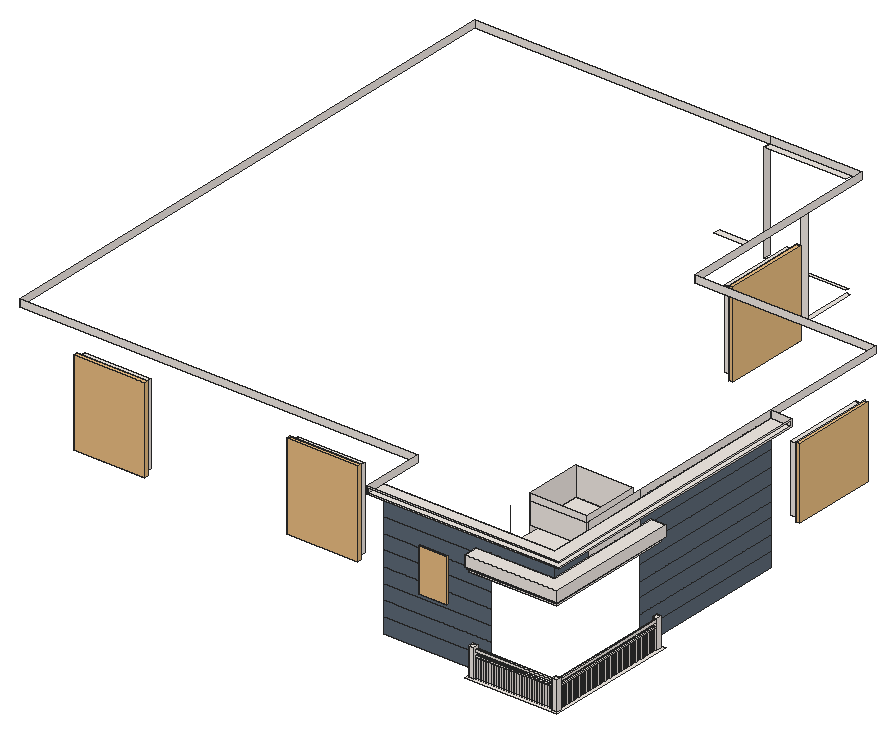
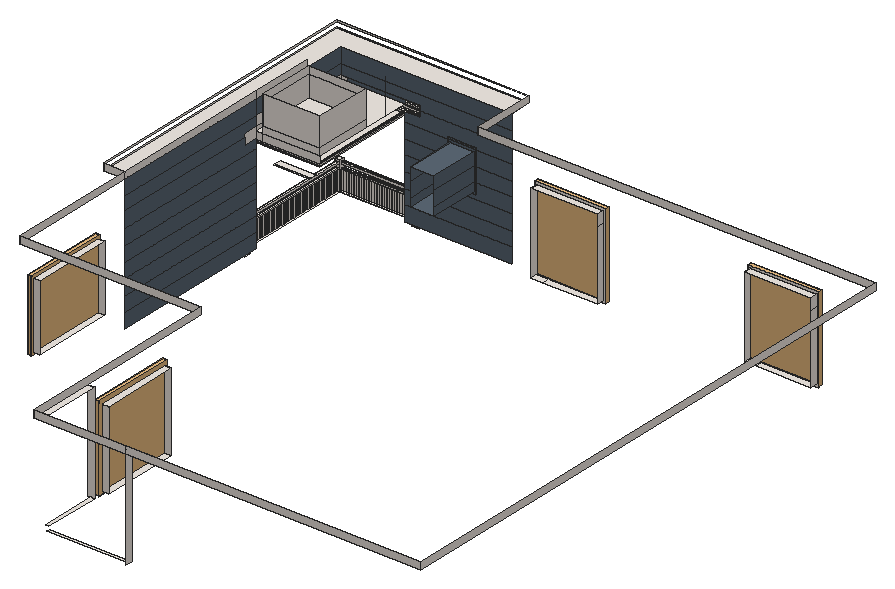
# SketchUp Ruby script. Lengths in inches.
U = 1.inch
M = Sketchup.active_model
def pt(a) = Geom::Point3d.new(a.map { |v| v * U })
def face(e, loops, mat)
  f = e.add_face(loops[0].map { |a| pt(a) })
  loops[1..].each { |l| e.add_face(l.map { |a| pt(a) }).erase! }
  f.material = f.back_material = mat if mat
  f
end
# faces: each face lists its corners as indices into pts; further lists are holes
def faces(e, pts, list, mat = nil) = list.each { |f| face(e, (f[0].is_a?(Array) ? f : [f]).map { |l| l.map { |i| pts[i] } }, mat) }
# xy, xz, yz: faces in a plane at the given z, y or x. An outline is a flat list of corners, or four numbers for a rectangle; further outlines are holes
def ring(l) = l.size == 4 ? [[l[0], l[1]], [l[2], l[1]], [l[2], l[3]], [l[0], l[3]]] : l.each_slice(2).to_a
def flat(e, list, mat, &to3) = list.each { |f| face(e, (f[0].is_a?(Array) ? f : [f]).map { |l| ring(l).map { |u, v| to3.(u, v) } }, mat) }
def xy(e, z, list, mat = nil) = flat(e, list, mat) { |x, y| [x, y, z] }
def xz(e, y, list, mat = nil) = flat(e, list, mat) { |x, z| [x, y, z] }
def yz(e, x, list, mat = nil) = flat(e, list, mat) { |y, z| [x, y, z] }
def lines(e, pts, list) = list.each { |a, b| e.add_line(pt(pts[a]), pt(pts[b])) }
# prism: a flat outline (further loops are holes) pulled along v
def prism(e, loops, v, mat = nil)
  f = face(e, loops, mat); d = Geom::Vector3d.new(v.map { |x| x * U })
  f.pushpull(f.normal.samedirection?(d) ? d.length : -d.length)
end
def box(e, o, s, mat = nil) = prism(e, [[o, [o[0] + s[0], o[1], o[2]], [o[0] + s[0], o[1] + s[1], o[2]], [o[0], o[1] + s[1], o[2]]]], [0, 0, s[2]], mat)
def at(x, y, z, deg = 0) = Geom::Transformation.translation(pt([x, y, z])) * Geom::Transformation.rotation(ORIGIN, Z_AXIS, deg.degrees)
def axes(o, x, y, z) = Geom::Transformation.new([*x, 0, *y, 0, *z, 0, *pt(o).to_a, 1])
def part(name) = M.definitions.add(name)
# library, detail: a bought-in or finely detailed component or shape, given as its bounding box
def library(name, o, s) = part(name).tap { |d| box(d.entities, o, s) }
def detail(e, o, s) = box(e.add_group.entities, o, s)
def put(e, d, t, mat = nil) = e.add_instance(d, t).tap { |i| i.material = mat if mat }
def group(e, t, mat = nil) = e.add_group.tap { |g| g.transformation = t; g.material = mat if mat }.entities
root = M.entities
M.materials.add("D01_Frost_White").color = [242, 235, 229]
M.materials.add("Denim_03_1K").color = [93, 106, 119]
c1 = library("mesh-163",[-551.08,-704.17,-20.03],[1929.24,1401.85,86.96])
c2 = part("Group11")
put(c2.entities,c1,at(0,0,0))
xy(root,258,[[[426,6,504,6,504,120,492,120,492,114,498,114,498,12,432,12,432,18,426,18],[498,8,502,12],[498,114,502,118],[428,8,432,12],[477.804,9.471,478.204,10.971],[475.655,9.471,476.055,10.971],[473.505,9.471,473.905,10.971],[471.356,9.471,471.756,10.971],[469.206,9.471,469.606,10.971],[467.057,9.471,467.457,10.971],[464.908,9.471,465.308,10.971],[462.758,9.471,463.158,10.971],[460.609,9.471,461.009,10.971],[458.459,9.471,458.859,10.971],[456.31,9.471,456.71,10.971],[454.16,9.471,454.56,10.971],[452.011,9.471,452.411,10.971],[449.862,9.471,450.262,10.971],[447.712,9.471,448.112,10.971],[445.563,9.471,445.963,10.971],[443.413,9.471,443.813,10.971],[441.264,9.471,441.664,10.971],[439.115,9.471,439.515,10.971],[432.666,9.471,433.066,10.971],[434.816,9.471,435.216,10.971],[436.965,9.471,437.365,10.971],[499.533,113.2,500.936,113.6],[499.533,110.689,500.936,111.089],[499.533,108.177,500.936,108.577],[499.533,105.666,500.936,106.066],[499.533,100.643,500.936,101.043],[499.533,103.154,500.936,103.554],[499.533,98.131,500.936,98.531]]],"D01_Frost_White")
xy(root,258.028,[[479.954,9.471,480.354,10.971],[482.103,9.471,482.503,10.971],[484.252,9.471,484.652,10.971],[486.402,9.471,486.802,10.971],[488.551,9.471,488.951,10.971],
  [490.701,9.471,491.101,10.971],[492.85,9.471,493.25,10.971],[495,9.471,495.4,10.971],[497.149,9.471,497.549,10.971],[499.533,12.739,500.936,13.139],
  [499.533,15.251,500.936,15.651],[499.533,17.762,500.936,18.162],[499.533,20.274,500.936,20.674],[499.533,22.785,500.936,23.185],[499.533,25.297,500.936,25.697],
  [499.533,27.808,500.936,28.208],[499.533,30.32,500.936,30.72],[499.533,32.831,500.936,33.231],[499.533,35.343,500.936,35.743],[499.533,37.854,500.936,38.254],
  [499.533,40.366,500.936,40.766],[499.533,42.877,500.936,43.277],[499.533,45.389,500.936,45.789],[499.533,47.9,500.936,48.3],[499.533,50.412,500.936,50.812],
  [499.533,52.923,500.936,53.323],[499.533,55.435,500.936,55.835],[499.533,57.947,500.936,58.347],[499.533,60.458,500.936,60.858],[499.533,62.97,500.936,63.37],
  [499.533,65.481,500.936,65.881],[499.533,67.993,500.936,68.393],[499.533,70.504,500.936,70.904],[499.533,73.016,500.936,73.416],[499.533,75.527,500.936,75.927],
  [499.533,78.039,500.936,78.439],[499.533,80.55,500.936,80.95],[499.533,83.062,500.936,83.462],[499.533,85.573,500.936,85.973],[499.533,88.085,500.936,88.485],
  [499.533,90.596,500.936,90.996],[499.533,93.108,500.936,93.508],[499.533,95.619,500.936,96.019]],"D01_Frost_White")
xy(root,274.664,[[[432,9.204,498,11.204],[432.666,9.471,433.066,10.971],[434.816,9.471,435.216,10.971],[436.965,9.471,437.365,10.971],[439.115,9.471,439.515,10.971],[441.264,9.471,441.664,10.971],[443.413,9.471,443.813,10.971],[445.563,9.471,445.963,10.971],[447.712,9.471,448.112,10.971],[449.862,9.471,450.262,10.971],[452.011,9.471,452.411,10.971],[454.16,9.471,454.56,10.971],[456.31,9.471,456.71,10.971],[458.459,9.471,458.859,10.971],[460.609,9.471,461.009,10.971],[462.758,9.471,463.158,10.971],[464.908,9.471,465.308,10.971],[467.057,9.471,467.457,10.971],[469.206,9.471,469.606,10.971],[471.356,9.471,471.756,10.971],[473.505,9.471,473.905,10.971],[475.655,9.471,476.055,10.971],[477.804,9.471,478.204,10.971],[479.954,9.471,480.354,10.971],[482.103,9.471,482.503,10.971],[484.252,9.471,484.652,10.971],[486.402,9.471,486.802,10.971],[488.551,9.471,488.951,10.971],[490.701,9.471,491.101,10.971],[492.85,9.471,493.25,10.971],[495,9.471,495.4,10.971],[497.149,9.471,497.549,10.971]],[[499.158,12,501.158,114],[499.533,12.739,500.936,13.139],[499.533,15.251,500.936,15.651],[499.533,17.762,500.936,18.162],[499.533,20.274,500.936,20.674],[499.533,22.785,500.936,23.185],[499.533,25.297,500.936,25.697],[499.533,27.808,500.936,28.208],[499.533,30.32,500.936,30.72],[499.533,32.831,500.936,33.231],[499.533,35.343,500.936,35.743],[499.533,37.854,500.936,38.254],[499.533,40.366,500.936,40.766],[499.533,42.877,500.936,43.277],[499.533,45.389,500.936,45.789],[499.533,47.9,500.936,48.3],[499.533,50.412,500.936,50.812],[499.533,52.923,500.936,53.323],[499.533,55.435,500.936,55.835],[499.533,57.947,500.936,58.347],[499.533,60.458,500.936,60.858],[499.533,62.97,500.936,63.37],[499.533,65.481,500.936,65.881],[499.533,67.993,500.936,68.393],[499.533,70.504,500.936,70.904],[499.533,73.016,500.936,73.416],[499.533,75.527,500.936,75.927],[499.533,78.039,500.936,78.439],[499.533,80.55,500.936,80.95],[499.533,83.062,500.936,83.462],[499.533,85.573,500.936,85.973],[499.533,88.085,500.936,88.485],[499.533,90.596,500.936,90.996],[499.533,93.108,500.936,93.508],[499.533,95.619,500.936,96.019],[499.533,98.131,500.936,98.531],[499.533,100.643,500.936,101.043],[499.533,103.154,500.936,103.554],[499.533,105.666,500.936,106.066],[499.533,108.177,500.936,108.577],[499.533,110.689,500.936,111.089],[499.533,113.2,500.936,113.6]],[499.155,12.739,499.158,13.139]],"D01_Frost_White")
xy(root,275.664,[[432,9.204,498,11.204],[499.158,12,501.158,114]],"D01_Frost_White")
xy(root,278.282,[[432,9.204,498,11.204],[499.158,12,501.158,114]],"D01_Frost_White")
xy(root,280.282,[[432,9.204,498,11.204],[499.158,12,501.158,114]],"D01_Frost_White")
xy(root,282,[[428,8,432,12],[498,8,502,12],[498,114,502,118]],"D01_Frost_White")
xy(root,284,[[62,54,108,60],[108,54,118,60],[242,54,288,60],[288,54,298,60],[486,275,492,343]],"D01_Frost_White")
xy(root,285,[[333,396,339,462]],"D01_Frost_White")
xy(root,288,[[333,477,336,525],[261,528,330,531]],"D01_Frost_White")
xy(root,302,[[380,18,400,60]],"Denim_03_1K")
xy(root,332.2,[[380,18,400,60]],"Denim_03_1K")
xy(root,333,[[441,108,471,114],[441,114,471,115.5],[264,471,294,477]],"D01_Frost_White")
xy(root,336,[[[444,12,498,102],[486,21.031,492,60]],[486,21.031,492,54],[486,29.003,492,60]],"D01_Frost_White")
xy(root,338,[[[428,8,428,16,440,16,440,106,494,106,494,118,502,118,502,8],[430,10,500,10,500,116,496,116,496,104,442,104,442,14,430,14]],[[430,10,430,14,442,14,442,104,496,104,496,116,500,116,500,10],[444,12,498,102]]],"D01_Frost_White")
xy(root,340,[[[427,7,427,17,439,17,439,107,493,107,493,119,503,119,503,7],[428,8,502,8,502,118,494,118,494,106,440,106,440,16,428,16]],[486,275,492,343]],"D01_Frost_White")
xy(root,342,[[[426,6,426,18,438,18,438,108,492,108,492,120,504,120,504,6],[427,7,503,7,503,119,493,119,493,107,439,107,439,17,427,17]],[486,54,492,60]],"D01_Frost_White")
xy(root,348,[[438,18,438,108,492,108,492,60,486,60,486,18],[486,18,492,54],[486,54,492,60]],"D01_Frost_White")
xy(root,351,[[426,6,504,6,504,120,492,120,492,18,426,18],[333,396,339,462]],"D01_Frost_White")
xy(root,352,[[62,54,118,60],[242,54,298,60]],"D01_Frost_White")
xy(root,354,[[438,60,486,108]],"D01_Frost_White")
xy(root,372,[[348,0,348,18,492,18,492,246,510,246,510,0],[333,477,339,525],[261,528,330,534]],"D01_Frost_White")
xz(root,0,[[348,372,510,372,510,373,349,373,349,377,510,377,510,378,348,378]],"D01_Frost_White")
xz(root,6,[[426,342,504,351]],"D01_Frost_White")
xz(root,7,[[427,340,503,342]],"D01_Frost_White")
xz(root,8,[[428,258,432,282],[498,258,502,282],[428,338,502,340]],"D01_Frost_White")
xz(root,9.204,[[432,274.664,498,275.664],[432,278.282,498,280.282]],"D01_Frost_White")
xz(root,9.471,[[432.666,258,433.066,274.664],[434.816,258,435.216,274.664],[436.965,258,437.365,274.664],[439.115,258,439.515,274.664],[441.264,258,441.664,274.664],
  [443.413,258,443.813,274.664],[445.563,258,445.963,274.664],[447.712,258,448.112,274.664],[449.862,258,450.262,274.664],[452.011,258,452.411,274.664],
  [454.16,258,454.56,274.664],[456.31,258,456.71,274.664],[458.459,258,458.859,274.664],[460.609,258,461.009,274.664],[462.758,258,463.158,274.664],
  [464.908,258,465.308,274.664],[467.057,258,467.457,274.664],[469.206,258,469.606,274.664],[471.356,258,471.756,274.664],[473.505,258,473.905,274.664],
  [475.655,258,476.055,274.664],[477.804,258,478.204,274.664],[479.954,258.028,480.354,274.664],[482.103,258.028,482.503,274.664],[484.252,258.028,484.652,274.664],
  [486.402,258.028,486.802,274.664],[488.551,258.028,488.951,274.664],[490.701,258.028,491.101,274.664],[492.85,258.028,493.25,274.664],[495,258.028,495.4,274.664],
  [497.149,258.028,497.549,274.664]],"D01_Frost_White")
xz(root,10.971,[[432.666,258,433.066,274.664],[434.816,258,435.216,274.664],[436.965,258,437.365,274.664],[439.115,258,439.515,274.664],[441.264,258,441.664,274.664],
  [443.413,258,443.813,274.664],[445.563,258,445.963,274.664],[447.712,258,448.112,274.664],[449.862,258,450.262,274.664],[452.011,258,452.411,274.664],
  [454.16,258,454.56,274.664],[456.31,258,456.71,274.664],[458.459,258,458.859,274.664],[460.609,258,461.009,274.664],[462.758,258,463.158,274.664],
  [464.908,258,465.308,274.664],[467.057,258,467.457,274.664],[469.206,258,469.606,274.664],[471.356,258,471.756,274.664],[473.505,258,473.905,274.664],
  [475.655,258,476.055,274.664],[477.804,258,478.204,274.664],[479.954,258.028,480.354,274.664],[482.103,258.028,482.503,274.664],[484.252,258.028,484.652,274.664],
  [486.402,258.028,486.802,274.664],[488.551,258.028,488.951,274.664],[490.701,258.028,491.101,274.664],[492.85,258.028,493.25,274.664],[495,258.028,495.4,274.664],
  [497.149,258.028,497.549,274.664]],"D01_Frost_White")
xz(root,11.204,[[432,274.664,498,275.664],[432,278.282,498,280.282]],"D01_Frost_White")
xz(root,12,[[428,258,432,282],[498,258,498,275.664,499.158,275.664,499.158,274.664,501.158,274.664,501.158,280.282,498,280.282,498,282,502,282,502,258],[498,275.664,498,280.282,499.158,280.282,499.158,278.282,501.158,278.282,501.158,275.664],[444,336,498,338]],"D01_Frost_White")
xz(root,12.739,[[499.533,258.028,500.936,274.664]],"D01_Frost_White")
xz(root,13.139,[[499.533,258.028,500.936,274.664]],"D01_Frost_White")
xz(root,15.251,[[499.533,258.028,500.936,274.664]],"D01_Frost_White")
xz(root,15.651,[[499.533,258.028,500.936,274.664]],"D01_Frost_White")
xz(root,16,[[428,338,440,340]],"D01_Frost_White")
xz(root,17,[[427,340,439,342]],"D01_Frost_White")
xz(root,17.762,[[499.533,258.028,500.936,274.664]],"D01_Frost_White")
xz(root,18,[[486,348,492,351]],"D01_Frost_White")
xz(root,18,[[348,258.6,438,271.2],[348,271.2,438,283.8],[348,283.8,438,296.4],[348,296.4,438,296.4,438,309,402,309,402,300,378,300,378,309,348,309],[[378,300,402,334.2],[380,302,400,332.2]],
  [348,309,378,321.6],[402,309,438,321.6],[348,321.6,378,334.2],[402,321.6,438,334.2],[348,334.2,378,334.2,378,336,402,336,402,334.2,438,334.2,438,342,426,342,426,346.8,348,346.8],
  [378,334.2,402,336],[348,346.8,426,346.8,426,351,492,351,492,359.4,348,359.4],[438,348,486,351],[348,359.4,492,372]],"Denim_03_1K")
xz(root,18.162,[[499.533,258.028,500.936,274.664]],"D01_Frost_White")
xz(root,20.274,[[499.533,258.028,500.936,274.664]],"D01_Frost_White")
xz(root,20.674,[[499.533,258.028,500.936,274.664]],"D01_Frost_White")
xz(root,22.785,[[499.533,258.028,500.936,274.664]],"D01_Frost_White")
xz(root,23.185,[[499.533,258.028,500.936,274.664]],"D01_Frost_White")
xz(root,25.297,[[499.533,258.028,500.936,274.664]],"D01_Frost_White")
xz(root,25.697,[[499.533,258.028,500.936,274.664]],"D01_Frost_White")
xz(root,27.808,[[499.533,258.028,500.936,274.664]],"D01_Frost_White")
xz(root,28.208,[[499.533,258.028,500.936,274.664]],"D01_Frost_White")
xz(root,30.32,[[499.533,258.028,500.936,274.664]],"D01_Frost_White")
xz(root,30.72,[[499.533,258.028,500.936,274.664]],"D01_Frost_White")
xz(root,32.831,[[499.533,258.028,500.936,274.664]],"D01_Frost_White")
xz(root,33.231,[[499.533,258.028,500.936,274.664]],"D01_Frost_White")
xz(root,35.343,[[499.533,258.028,500.936,274.664]],"D01_Frost_White")
xz(root,35.743,[[499.533,258.028,500.936,274.664]],"D01_Frost_White")
xz(root,37.854,[[499.533,258.028,500.936,274.664]],"D01_Frost_White")
xz(root,38.254,[[499.533,258.028,500.936,274.664]],"D01_Frost_White")
xz(root,40.366,[[499.533,258.028,500.936,274.664]],"D01_Frost_White")
xz(root,40.766,[[499.533,258.028,500.936,274.664]],"D01_Frost_White")
xz(root,42.877,[[499.533,258.028,500.936,274.664]],"D01_Frost_White")
xz(root,43.277,[[499.533,258.028,500.936,274.664]],"D01_Frost_White")
xz(root,45.389,[[499.533,258.028,500.936,274.664]],"D01_Frost_White")
xz(root,45.789,[[499.533,258.028,500.936,274.664]],"D01_Frost_White")
xz(root,47.9,[[499.533,258.028,500.936,274.664]],"D01_Frost_White")
xz(root,48.3,[[499.533,258.028,500.936,274.664]],"D01_Frost_White")
xz(root,50.412,[[499.533,258.028,500.936,274.664]],"D01_Frost_White")
xz(root,50.812,[[499.533,258.028,500.936,274.664]],"D01_Frost_White")
xz(root,52.923,[[499.533,258.028,500.936,274.664]],"D01_Frost_White")
xz(root,53.323,[[499.533,258.028,500.936,274.664]],"D01_Frost_White")
xz(root,54,[[[60,282,120,354],[62,284,118,352]],[[240,282,300,354],[242,284,298,352]],[486,336,492,342],[486,342,492,348],[12,372,348,378]],"D01_Frost_White")
xz(root,55.435,[[499.533,258.028,500.936,274.664]],"D01_Frost_White")
xz(root,55.835,[[499.533,258.028,500.936,274.664]],"D01_Frost_White")
xz(root,57.947,[[499.533,258.028,500.936,274.664]],"D01_Frost_White")
xz(root,58.347,[[499.533,258.028,500.936,274.664]],"D01_Frost_White")
xz(root,60,[[486,336,492,342],[486,342,492,348],[438,354,486,372],[438,372,486,378]],"D01_Frost_White")
xz(root,60.458,[[499.533,258.028,500.936,274.664]],"D01_Frost_White")
xz(root,60.858,[[499.533,258.028,500.936,274.664]],"D01_Frost_White")
xz(root,62.97,[[499.533,258.028,500.936,274.664]],"D01_Frost_White")
xz(root,63.37,[[499.533,258.028,500.936,274.664]],"D01_Frost_White")
xz(root,65.481,[[499.533,258.028,500.936,274.664]],"D01_Frost_White")
xz(root,65.881,[[499.533,258.028,500.936,274.664]],"D01_Frost_White")
xz(root,67.993,[[499.533,258.028,500.936,274.664]],"D01_Frost_White")
xz(root,68.393,[[499.533,258.028,500.936,274.664]],"D01_Frost_White")
xz(root,70.504,[[499.533,258.028,500.936,274.664]],"D01_Frost_White")
xz(root,70.904,[[499.533,258.028,500.936,274.664]],"D01_Frost_White")
xz(root,73.016,[[499.533,258.028,500.936,274.664]],"D01_Frost_White")
xz(root,73.416,[[499.533,258.028,500.936,274.664]],"D01_Frost_White")
xz(root,75.527,[[499.533,258.028,500.936,274.664]],"D01_Frost_White")
xz(root,75.927,[[499.533,258.028,500.936,274.664]],"D01_Frost_White")
xz(root,78.039,[[499.533,258.028,500.936,274.664]],"D01_Frost_White")
xz(root,78.439,[[499.533,258.028,500.936,274.664]],"D01_Frost_White")
xz(root,80.55,[[499.533,258.028,500.936,274.664]],"D01_Frost_White")
xz(root,80.95,[[499.533,258.028,500.936,274.664]],"D01_Frost_White")
xz(root,83.062,[[499.533,258.028,500.936,274.664]],"D01_Frost_White")
xz(root,83.462,[[499.533,258.028,500.936,274.664]],"D01_Frost_White")
xz(root,85.573,[[499.533,258.028,500.936,274.664]],"D01_Frost_White")
xz(root,85.973,[[499.533,258.028,500.936,274.664]],"D01_Frost_White")
xz(root,88.085,[[499.533,258.028,500.936,274.664]],"D01_Frost_White")
xz(root,88.485,[[499.533,258.028,500.936,274.664]],"D01_Frost_White")
xz(root,90.596,[[499.533,258.028,500.936,274.664]],"D01_Frost_White")
xz(root,90.996,[[499.533,258.028,500.936,274.664]],"D01_Frost_White")
xz(root,93.108,[[499.533,258.028,500.936,274.664]],"D01_Frost_White")
xz(root,93.508,[[499.533,258.028,500.936,274.664]],"D01_Frost_White")
xz(root,95.619,[[499.533,258.028,500.936,274.664]],"D01_Frost_White")
xz(root,96.019,[[499.533,258.028,500.936,274.664]],"D01_Frost_White")
xz(root,98.131,[[499.533,258,500.936,274.664]],"D01_Frost_White")
xz(root,98.531,[[499.533,258,500.936,274.664]],"D01_Frost_White")
xz(root,100.643,[[499.533,258,500.936,274.664]],"D01_Frost_White")
xz(root,101.043,[[499.533,258,500.936,274.664]],"D01_Frost_White")
xz(root,102,[[444,336,486,338],[486,336,498,338]],"D01_Frost_White")
xz(root,103.154,[[499.533,258,500.936,274.664]],"D01_Frost_White")
xz(root,103.554,[[499.533,258,500.936,274.664]],"D01_Frost_White")
xz(root,105.666,[[499.533,258,500.936,274.664]],"D01_Frost_White")
xz(root,106,[[440,338,486,340],[486,338,494,340]],"D01_Frost_White")
xz(root,106.066,[[499.533,258,500.936,274.664]],"D01_Frost_White")
xz(root,107,[[439,340,486,342],[486,340,493,342]],"D01_Frost_White")
xz(root,108,[[438,342,486,348],[486,342,492,348],[438,348,486,354],[438,354,486,378]],"D01_Frost_White")
xz(root,108.177,[[499.533,258,500.936,274.664]],"D01_Frost_White")
xz(root,108.577,[[499.533,258,500.936,274.664]],"D01_Frost_White")
xz(root,110.689,[[499.533,258,500.936,274.664]],"D01_Frost_White")
xz(root,111.089,[[499.533,258,500.936,274.664]],"D01_Frost_White")
xz(root,113.2,[[499.533,258,500.936,274.664]],"D01_Frost_White")
xz(root,113.6,[[499.533,258,500.936,274.664]],"D01_Frost_White")
xz(root,114,[[[498,258,502,282],[499.158,278.282,501.158,280.282],[499.158,274.664,501.158,275.664]]],"D01_Frost_White")
xz(root,118,[[498,258,502,282],[494,338,502,340]],"D01_Frost_White")
xz(root,119,[[493,340,503,342]],"D01_Frost_White")
xz(root,120,[[492,342,504,351]],"D01_Frost_White")
xz(root,246,[[492,372,510,378]],"D01_Frost_White")
xz(root,275,[[486,284,492,340]],"D01_Frost_White")
xz(root,343,[[486,284,492,340]],"D01_Frost_White")
xz(root,357,[[339,372,492,378]],"D01_Frost_White")
xz(root,396,[[333,285,339,351]],"D01_Frost_White")
xz(root,462,[[333,285,339,351]],"D01_Frost_White")
xz(root,477,[[333,288,339,372]],"D01_Frost_White")
xz(root,534,[[12,372,261,378],[261,372,339,378]],"D01_Frost_White")
yz(root,12,[[54,372,534,378]],"D01_Frost_White")
yz(root,62,[[54,284,60,342],[54,342,60,352]],"D01_Frost_White")
yz(root,118,[[54,284,60,352]],"D01_Frost_White")
yz(root,242,[[54,284,60,342],[54,342,60,352]],"D01_Frost_White")
yz(root,261,[[528,288,534,372]],"D01_Frost_White")
yz(root,298,[[54,284,60,352]],"D01_Frost_White")
yz(root,339,[[[393,282,465,354],[396,285,462,351]],[357,372,534,378]],"D01_Frost_White")
yz(root,348,[[0,372,54,378]],"D01_Frost_White")
yz(root,380,[[18,302,60,309],[18,309,60,321.6],[18,321.6,60,332.2]],"Denim_03_1K")
yz(root,400,[[18,302,60,309],[18,309,60,321.6],[18,321.6,60,332.2]],"Denim_03_1K")
yz(root,426,[[6,342,18,346.8],[6,346.8,18,351]],"D01_Frost_White")
yz(root,427,[[7,340,17,342]],"D01_Frost_White")
yz(root,428,[[8,258,12,282],[8,338,16,340]],"D01_Frost_White")
yz(root,432,[[[8,258,12,282],[9.204,278.282,11.204,280.282],[9.204,274.664,11.204,275.664]]],"D01_Frost_White")
yz(root,432.666,[[9.471,258,10.971,274.664]],"D01_Frost_White")
yz(root,433.066,[[9.471,258,10.971,274.664]],"D01_Frost_White")
yz(root,434.816,[[9.471,258,10.971,274.664]],"D01_Frost_White")
yz(root,435.216,[[9.471,258,10.971,274.664]],"D01_Frost_White")
yz(root,436.965,[[9.471,258,10.971,274.664]],"D01_Frost_White")
yz(root,437.365,[[9.471,258,10.971,274.664]],"D01_Frost_White")
yz(root,438,[[60,348,108,354],[60,354,108,378]],"D01_Frost_White")
yz(root,439,[[17,340,107,342]],"D01_Frost_White")
yz(root,439.115,[[9.471,258,10.971,274.664]],"D01_Frost_White")
yz(root,439.515,[[9.471,258,10.971,274.664]],"D01_Frost_White")
yz(root,440,[[16,338,106,340]],"D01_Frost_White")
yz(root,441.264,[[9.471,258,10.971,274.664]],"D01_Frost_White")
yz(root,441.664,[[9.471,258,10.971,274.664]],"D01_Frost_White")
yz(root,443.413,[[9.471,258,10.971,274.664]],"D01_Frost_White")
yz(root,443.813,[[9.471,258,10.971,274.664]],"D01_Frost_White")
yz(root,444,[[12,336,102,338]],"D01_Frost_White")
yz(root,445.563,[[9.471,258,10.971,274.664]],"D01_Frost_White")
yz(root,445.963,[[9.471,258,10.971,274.664]],"D01_Frost_White")
yz(root,447.712,[[9.471,258,10.971,274.664]],"D01_Frost_White")
yz(root,448.112,[[9.471,258,10.971,274.664]],"D01_Frost_White")
yz(root,449.862,[[9.471,258,10.971,274.664]],"D01_Frost_White")
yz(root,450.262,[[9.471,258,10.971,274.664]],"D01_Frost_White")
yz(root,452.011,[[9.471,258,10.971,274.664]],"D01_Frost_White")
yz(root,452.411,[[9.471,258,10.971,274.664]],"D01_Frost_White")
yz(root,454.16,[[9.471,258,10.971,274.664]],"D01_Frost_White")
yz(root,454.56,[[9.471,258,10.971,274.664]],"D01_Frost_White")
yz(root,456.31,[[9.471,258,10.971,274.664]],"D01_Frost_White")
yz(root,456.71,[[9.471,258,10.971,274.664]],"D01_Frost_White")
yz(root,458.459,[[9.471,258,10.971,274.664]],"D01_Frost_White")
yz(root,458.859,[[9.471,258,10.971,274.664]],"D01_Frost_White")
yz(root,460.609,[[9.471,258,10.971,274.664]],"D01_Frost_White")
yz(root,461.009,[[9.471,258,10.971,274.664]],"D01_Frost_White")
yz(root,462.758,[[9.471,258,10.971,274.664]],"D01_Frost_White")
yz(root,463.158,[[9.471,258,10.971,274.664]],"D01_Frost_White")
yz(root,464.908,[[9.471,258,10.971,274.664]],"D01_Frost_White")
yz(root,465.308,[[9.471,258,10.971,274.664]],"D01_Frost_White")
yz(root,467.057,[[9.471,258,10.971,274.664]],"D01_Frost_White")
yz(root,467.457,[[9.471,258,10.971,274.664]],"D01_Frost_White")
yz(root,469.206,[[9.471,258,10.971,274.664]],"D01_Frost_White")
yz(root,469.606,[[9.471,258,10.971,274.664]],"D01_Frost_White")
yz(root,471.356,[[9.471,258,10.971,274.664]],"D01_Frost_White")
yz(root,471.756,[[9.471,258,10.971,274.664]],"D01_Frost_White")
yz(root,473.505,[[9.471,258,10.971,274.664]],"D01_Frost_White")
yz(root,473.905,[[9.471,258,10.971,274.664]],"D01_Frost_White")
yz(root,475.655,[[9.471,258,10.971,274.664]],"D01_Frost_White")
yz(root,476.055,[[9.471,258,10.971,274.664]],"D01_Frost_White")
yz(root,477.804,[[9.471,258,10.971,274.664]],"D01_Frost_White")
yz(root,478.204,[[9.471,258,10.971,274.664]],"D01_Frost_White")
yz(root,479.954,[[9.471,258.028,10.971,274.664]],"D01_Frost_White")
yz(root,480.354,[[9.471,258.028,10.971,274.664]],"D01_Frost_White")
yz(root,482.103,[[9.471,258.028,10.971,274.664]],"D01_Frost_White")
yz(root,482.503,[[9.471,258.028,10.971,274.664]],"D01_Frost_White")
yz(root,484.252,[[9.471,258.028,10.971,274.664]],"D01_Frost_White")
yz(root,484.652,[[9.471,258.028,10.971,274.664]],"D01_Frost_White")
yz(root,486,[[54,336,60,342],[54,342,60,348],[60,354,108,372],[60,372,108,378]],"D01_Frost_White")
yz(root,486.402,[[9.471,258.028,10.971,274.664]],"D01_Frost_White")
yz(root,486.802,[[9.471,258.028,10.971,274.664]],"D01_Frost_White")
yz(root,488.551,[[9.471,258.028,10.971,274.664]],"D01_Frost_White")
yz(root,488.951,[[9.471,258.028,10.971,274.664]],"D01_Frost_White")
yz(root,490.701,[[9.471,258.028,10.971,274.664]],"D01_Frost_White")
yz(root,491.101,[[9.471,258.028,10.971,274.664]],"D01_Frost_White")
yz(root,492,[[[273,282,345,342],[275,284,343,340]],[54,336,60,342],[54,342,60,348],[108,342,120,351],[18,348,54,351],
  [54,348,60,351],[60,348,108,351],[54,351,108,359.4],[54,372,108,378],[108,372,246,378],
  [246,372,357,378]],"D01_Frost_White")
yz(root,492,[[108,258.6,246,271.2],[108,271.2,246,283.8],[108,283.8,246,296.4],[108,296.4,246,309],[108,309,246,321.6],
  [108,321.6,246,334.2],[108,334.2,246,334.2,246,348,120,348,120,342,108,342],[120,348,246,348,246,359.4,108,359.4,108,351,120,351],[18,351,54,359.4],[18,359.4,54,372],
  [54,359.4,108,372],[108,359.4,246,372]],"Denim_03_1K")
yz(root,492.85,[[9.471,258.028,10.971,274.664]],"D01_Frost_White")
yz(root,493,[[107,340,119,342]],"D01_Frost_White")
yz(root,493.25,[[9.471,258.028,10.971,274.664]],"D01_Frost_White")
yz(root,494,[[106,338,118,340]],"D01_Frost_White")
yz(root,495,[[9.471,258.028,10.971,274.664]],"D01_Frost_White")
yz(root,495.4,[[9.471,258.028,10.971,274.664]],"D01_Frost_White")
yz(root,497.149,[[9.471,258.028,10.971,274.664]],"D01_Frost_White")
yz(root,497.549,[[9.471,258.028,10.971,274.664]],"D01_Frost_White")
yz(root,498,[[8,258,8,282,12,282,12,280.282,9.204,280.282,9.204,278.282,11.204,278.282,11.204,275.664,9.204,275.664,9.204,274.664,11.204,274.664,11.204,280.282,12,280.282,12,258],[114,258,118,282],[12,336,102,338]],"D01_Frost_White")
yz(root,499.158,[[12,274.664,114,275.664],[12,278.282,114,280.282]],"D01_Frost_White")
yz(root,499.533,[[98.131,258,98.531,274.664],[100.643,258,101.043,274.664],[103.154,258,103.554,274.664],[105.666,258,106.066,274.664],[108.177,258,108.577,274.664],
  [110.689,258,111.089,274.664],[113.2,258,113.6,274.664],[12.739,258.028,13.139,274.664],[15.251,258.028,15.651,274.664],[17.762,258.028,18.162,274.664],
  [20.274,258.028,20.674,274.664],[22.785,258.028,23.185,274.664],[25.297,258.028,25.697,274.664],[27.808,258.028,28.208,274.664],[30.32,258.028,30.72,274.664],
  [32.831,258.028,33.231,274.664],[35.343,258.028,35.743,274.664],[37.854,258.028,38.254,274.664],[40.366,258.028,40.766,274.664],[42.877,258.028,43.277,274.664],
  [45.389,258.028,45.789,274.664],[47.9,258.028,48.3,274.664],[50.412,258.028,50.812,274.664],[52.923,258.028,53.323,274.664],[55.435,258.028,55.835,274.664],
  [57.947,258.028,58.347,274.664],[60.458,258.028,60.858,274.664],[62.97,258.028,63.37,274.664],[65.481,258.028,65.881,274.664],[67.993,258.028,68.393,274.664],
  [70.504,258.028,70.904,274.664],[73.016,258.028,73.416,274.664],[75.527,258.028,75.927,274.664],[78.039,258.028,78.439,274.664],[80.55,258.028,80.95,274.664],
  [83.062,258.028,83.462,274.664],[85.573,258.028,85.973,274.664],[88.085,258.028,88.485,274.664],[90.596,258.028,90.996,274.664],[93.108,258.028,93.508,274.664],
  [95.619,258.028,96.019,274.664]],"D01_Frost_White")
yz(root,500.936,[[98.131,258,98.531,274.664],[100.643,258,101.043,274.664],[103.154,258,103.554,274.664],[105.666,258,106.066,274.664],[108.177,258,108.577,274.664],
  [110.689,258,111.089,274.664],[113.2,258,113.6,274.664],[12.739,258.028,13.139,274.664],[15.251,258.028,15.651,274.664],[17.762,258.028,18.162,274.664],
  [20.274,258.028,20.674,274.664],[22.785,258.028,23.185,274.664],[25.297,258.028,25.697,274.664],[27.808,258.028,28.208,274.664],[30.32,258.028,30.72,274.664],
  [32.831,258.028,33.231,274.664],[35.343,258.028,35.743,274.664],[37.854,258.028,38.254,274.664],[40.366,258.028,40.766,274.664],[42.877,258.028,43.277,274.664],
  [45.389,258.028,45.789,274.664],[47.9,258.028,48.3,274.664],[50.412,258.028,50.812,274.664],[52.923,258.028,53.323,274.664],[55.435,258.028,55.835,274.664],
  [57.947,258.028,58.347,274.664],[60.458,258.028,60.858,274.664],[62.97,258.028,63.37,274.664],[65.481,258.028,65.881,274.664],[67.993,258.028,68.393,274.664],
  [70.504,258.028,70.904,274.664],[73.016,258.028,73.416,274.664],[75.527,258.028,75.927,274.664],[78.039,258.028,78.439,274.664],[80.55,258.028,80.95,274.664],
  [83.062,258.028,83.462,274.664],[85.573,258.028,85.973,274.664],[88.085,258.028,88.485,274.664],[90.596,258.028,90.996,274.664],[93.108,258.028,93.508,274.664],
  [95.619,258.028,96.019,274.664]],"D01_Frost_White")
yz(root,501.158,[[12,274.664,114,275.664],[12,278.282,114,280.282]],"D01_Frost_White")
yz(root,502,[[8,258,12,282],[114,258,118,282],[8,338,118,340]],"D01_Frost_White")
yz(root,503,[[7,340,119,342]],"D01_Frost_White")
yz(root,504,[[6,342,120,351]],"D01_Frost_White")
yz(root,510,[[0,372,246,372,246,378,0,378,0,377,245,377,245,373,0,373]],"D01_Frost_White")
p = [[438,39,348],[438,39,378],[486,60,348],[486,60,354],[438,18,346.8],[426,18,346.8]]
lines(root,p,[[0,1],[2,3],[4,5]])
put(root,c2,axes([257.14,53.21,318.02],[0.0311,0,0],[0,0,0.05157],[0,-0.03937,0]))
put(root,c2,axes([494.63,324,312.14],[0,-0.03701,0],[0,0,0.0428],[-0.03937,0,0]))
put(root,c2,axes([77.14,53.21,318.29],[0.0311,0,0],[0,0,0.05118],[0,-0.03937,0]))
put(root,c2,axes([341.63,444,318.29],[0,-0.03701,0],[0,0,0.05118],[-0.03937,0,0]))
put(root,c2,axes([384.83,17.76,318.04],[0.0124,0,0],[0,0,0.02575],[0,-0.01181,0]))
